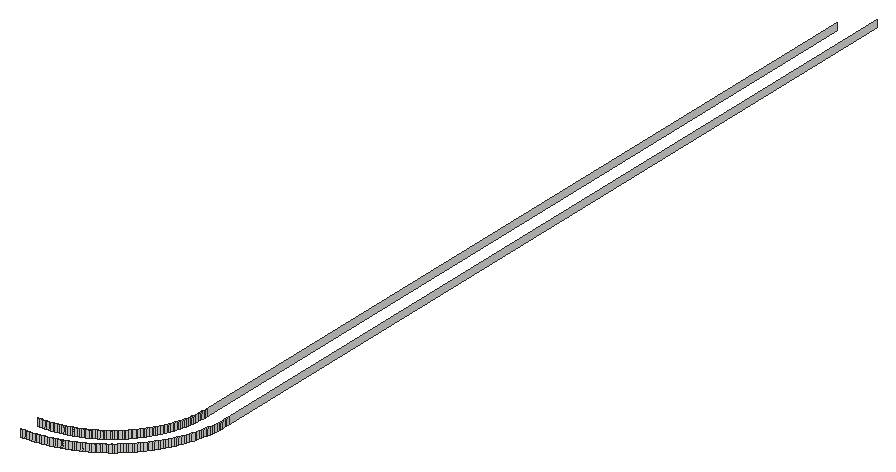
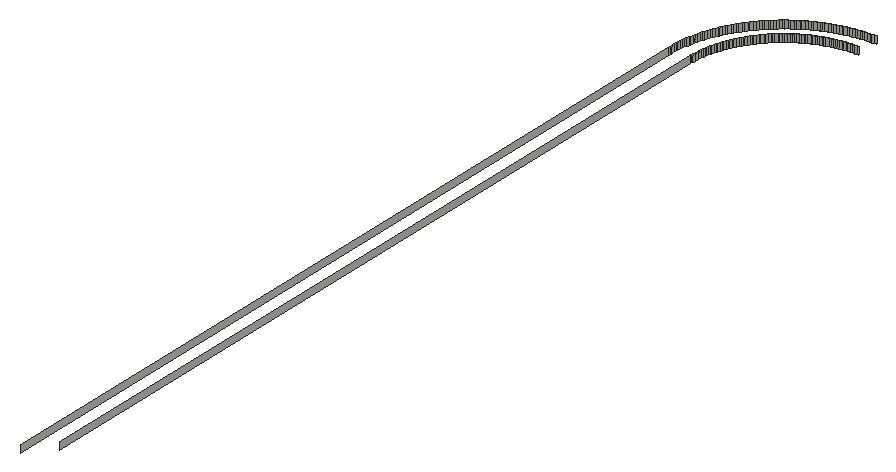
# SketchUp Ruby script. Lengths in inches.
U = 1.inch
M = Sketchup.active_model
def pt(a) = Geom::Point3d.new(a.map { |v| v * U })
def face(e, loops, mat)
  f = e.add_face(loops[0].map { |a| pt(a) })
  loops[1..].each { |l| e.add_face(l.map { |a| pt(a) }).erase! }
  f.material = f.back_material = mat if mat
  f
end
# faces: each face lists its corners as indices into pts; further lists are holes
def faces(e, pts, list, mat = nil) = list.each { |f| face(e, (f[0].is_a?(Array) ? f : [f]).map { |l| l.map { |i| pts[i] } }, mat) }
# xy, xz, yz: faces in a plane at the given z, y or x. An outline is a flat list of corners, or four numbers for a rectangle; further outlines are holes
def ring(l) = l.size == 4 ? [[l[0], l[1]], [l[2], l[1]], [l[2], l[3]], [l[0], l[3]]] : l.each_slice(2).to_a
def flat(e, list, mat, &to3) = list.each { |f| face(e, (f[0].is_a?(Array) ? f : [f]).map { |l| ring(l).map { |u, v| to3.(u, v) } }, mat) }
def xy(e, z, list, mat = nil) = flat(e, list, mat) { |x, y| [x, y, z] }
def xz(e, y, list, mat = nil) = flat(e, list, mat) { |x, z| [x, y, z] }
def yz(e, x, list, mat = nil) = flat(e, list, mat) { |y, z| [x, y, z] }
def lines(e, pts, list) = list.each { |a, b| e.add_line(pt(pts[a]), pt(pts[b])) }
# prism: a flat outline (further loops are holes) pulled along v
def prism(e, loops, v, mat = nil)
  f = face(e, loops, mat); d = Geom::Vector3d.new(v.map { |x| x * U })
  f.pushpull(f.normal.samedirection?(d) ? d.length : -d.length)
end
def box(e, o, s, mat = nil) = prism(e, [[o, [o[0] + s[0], o[1], o[2]], [o[0] + s[0], o[1] + s[1], o[2]], [o[0], o[1] + s[1], o[2]]]], [0, 0, s[2]], mat)
def at(x, y, z, deg = 0) = Geom::Transformation.translation(pt([x, y, z])) * Geom::Transformation.rotation(ORIGIN, Z_AXIS, deg.degrees)
def axes(o, x, y, z) = Geom::Transformation.new([*x, 0, *y, 0, *z, 0, *pt(o).to_a, 1])
def part(name) = M.definitions.add(name)
# library, detail: a bought-in or finely detailed component or shape, given as its bounding box
def library(name, o, s) = part(name).tap { |d| box(d.entities, o, s) }
def detail(e, o, s) = box(e.add_group.entities, o, s)
def put(e, d, t, mat = nil) = e.add_instance(d, t).tap { |i| i.material = mat if mat }
def group(e, t, mat = nil) = e.add_group.tap { |g| g.transformation = t; g.material = mat if mat }.entities
root = M.entities
xz(root,124,[[278,116,278.16,116.5]])
xz(root,124.01,[[278.3125,116,278.47,116.5]])
xz(root,125.5,[[278,116,278.13,116.5]])
xz(root,125.51,[[278.26,116,278.38,116.5]])
yz(root,284.49,[[131.62,116,131.74,116.5]])
yz(root,284.5,[[131.87,116,132,116.5],[132,116,186.5,116.5]])
yz(root,285.99,[[131.53,116,131.6875,116.5]])
yz(root,286,[[131.84,116,132,116.5],[132,116,188,116.5]])
p = [[278.3125,124.01,116],[278.16,124,116],[278.16,124,116.5],[278.3125,124.01,116.5],[278.63,124.02,116],[278.47,124.01,116],
  [278.47,124.01,116.5],[278.63,124.02,116.5],[278.78,124.04,116],[278.78,124.04,116.5],[278.94,124.06,116],[278.94,124.06,116.5],
  [279.1,124.08,116],[279.1,124.08,116.5],[279.25,124.1,116],[279.25,124.1,116.5],[279.41,124.125,116],[279.41,124.125,116.5],
  [279.5625,124.15,116],[279.5625,124.15,116.5],[279.71,124.1875,116],[279.71,124.1875,116.5],[279.87,124.22,116],[279.87,124.22,116.5],
  [280.02,124.26,116],[280.02,124.26,116.5],[280.17,124.3,116],[280.17,124.3,116.5],[280.32,124.34,116],[280.32,124.34,116.5],
  [280.47,124.39,116],[280.47,124.39,116.5],[280.62,124.44,116],[280.62,124.44,116.5],[280.77,124.49,116],[280.77,124.49,116.5],
  [280.92,124.55,116],[280.92,124.55,116.5],[281.0625,124.61,116],[281.0625,124.61,116.5],[281.21,124.67,116],[281.21,124.67,116.5],
  [281.35,124.73,116],[281.35,124.73,116.5],[281.49,124.8,116],[281.49,124.8,116.5],[281.63,124.87,116],[281.63,124.87,116.5],
  [281.77,124.94,116],[281.77,124.94,116.5],[281.91,125.02,116],[281.91,125.02,116.5],[282.05,125.1,116],[282.05,125.1,116.5],
  [282.18,125.18,116],[282.18,125.18,116.5],[282.3125,125.26,116],[282.3125,125.26,116.5],[282.44,125.35,116],[282.44,125.35,116.5],
  [282.57,125.4375,116],[282.57,125.4375,116.5],[282.7,125.53,116],[282.7,125.53,116.5],[278.13,125.5,116],[278.26,125.51,116],
  [278.26,125.51,116.5],[278.13,125.5,116.5],[278.38,125.51,116],[278.51,125.52,116],[278.51,125.52,116.5],[278.38,125.51,116.5],
  [278.64,125.53,116],[278.64,125.53,116.5],[278.76,125.55,116],[278.76,125.55,116.5],[278.89,125.5625,116],[278.89,125.5625,116.5],
  [282.83,125.62,116],[282.83,125.62,116.5],[279.02,125.58,116],[279.02,125.58,116.5],[279.14,125.6,116],[279.14,125.6,116.5],
  [279.27,125.625,116],[279.27,125.625,116.5],[279.39,125.65,116],[279.39,125.65,116.5],[282.95,125.72,116],[282.95,125.72,116.5],
  [279.52,125.68,116],[279.52,125.68,116.5],[279.64,125.71,116],[279.64,125.71,116.5],[279.76,125.74,116],[279.76,125.74,116.5],
  [279.89,125.78,116],[279.89,125.78,116.5],[283.08,125.82,116],[283.08,125.82,116.5],[280.01,125.82,116],[280.01,125.82,116.5],
  [280.13,125.86,116],[280.13,125.86,116.5],[283.2,125.92,116],[283.2,125.92,116.5],[280.25,125.9,116],[280.25,125.9,116.5],
  [280.37,125.95,116],[280.37,125.95,116.5],[280.49,125.99,116],[280.49,125.99,116.5],[283.3125,126.02,116],[283.3125,126.02,116.5],
  [280.6,126.04,116],[280.6,126.04,116.5],[280.72,126.1,116],[280.72,126.1,116.5],[283.43,126.125,116],[283.43,126.125,116.5],
  [280.84,126.15,116],[280.84,126.15,116.5],[283.54,126.23,116],[283.54,126.23,116.5],[280.95,126.21,116],[280.95,126.21,116.5],
  [281.0625,126.27,116],[281.0625,126.27,116.5],[283.66,126.34,116],[283.66,126.34,116.5],[281.18,126.33,116],[281.18,126.33,116.5],
  [281.29,126.39,116],[281.29,126.39,116.5],[283.77,126.46,116],[283.77,126.46,116.5],[281.4,126.46,116],[281.4,126.46,116.5],
  [281.5,126.53,116],[281.5,126.53,116.5],[281.61,126.6,116],[281.61,126.6,116.5],[283.875,126.57,116],[283.875,126.57,116.5],
  [281.72,126.67,116],[281.72,126.67,116.5],[283.98,126.6875,116],[283.98,126.6875,116.5],[281.82,126.74,116],[281.82,126.74,116.5],
  [281.92,126.82,116],[281.92,126.82,116.5],[284.08,126.8,116],[284.08,126.8,116.5],[282.02,126.9,116],[282.02,126.9,116.5],
  [284.18,126.92,116],[284.18,126.92,116.5],[282.125,126.98,116],[282.125,126.98,116.5],[284.28,127.05,116],[284.28,127.05,116.5],
  [282.22,127.06,116],[282.22,127.06,116.5],[284.38,127.17,116],[284.38,127.17,116.5],[282.32,127.14,116],[282.32,127.14,116.5],
  [282.41,127.23,116],[282.41,127.23,116.5],[282.5,127.3125,116],[282.5,127.3125,116.5],[284.47,127.3,116],[284.47,127.3,116.5],
  [282.6,127.4,116],[282.6,127.4,116.5],[284.5625,127.43,116],[284.5625,127.43,116.5],[282.69,127.49,116],[282.69,127.49,116.5],
  [284.65,127.56,116],[284.65,127.56,116.5],[282.77,127.59,116],[282.77,127.59,116.5],[282.86,127.68,116],[282.86,127.68,116.5],
  [284.74,127.6875,116],[284.74,127.6875,116.5],[282.94,127.78,116],[282.94,127.78,116.5],[284.82,127.82,116],[284.82,127.82,116.5],
  [283.02,127.875,116],[283.02,127.875,116.5],[284.9,127.95,116],[284.9,127.95,116.5],[283.1,127.98,116],[283.1,127.98,116.5],
  [283.18,128.08,116],[283.18,128.08,116.5],[284.98,128.09,116],[284.98,128.09,116.5],[283.26,128.18,116],[283.26,128.18,116.5],
  [285.06,128.23,116],[285.06,128.23,116.5],[283.33,128.28,116],[283.33,128.28,116.5],[285.13,128.37,116],[285.13,128.37,116.5],
  [283.4,128.39,116],[283.4,128.39,116.5],[283.47,128.5,116],[283.47,128.5,116.5],[285.2,128.51,116],[285.2,128.51,116.5],
  [283.54,128.6,116],[283.54,128.6,116.5],[285.27,128.65,116],[285.27,128.65,116.5],[283.61,128.71,116],[283.61,128.71,116.5],
  [283.67,128.82,116],[283.67,128.82,116.5],[285.33,128.79,116],[285.33,128.79,116.5],[283.73,128.9375,116],[283.73,128.9375,116.5],
  [285.39,128.9375,116],[285.39,128.9375,116.5],[283.79,129.05,116],[283.79,129.05,116.5],[285.45,129.08,116],[285.45,129.08,116.5],
  [283.85,129.16,116],[283.85,129.16,116.5],[285.51,129.23,116],[285.51,129.23,116.5],[283.9,129.28,116],[283.9,129.28,116.5],
  [285.56,129.38,116],[285.56,129.38,116.5],[283.96,129.4,116],[283.96,129.4,116.5],[284.01,129.51,116],[284.01,129.51,116.5],
  [285.61,129.53,116],[285.61,129.53,116.5],[284.05,129.63,116],[284.05,129.63,116.5],[285.66,129.68,116],[285.66,129.68,116.5],
  [284.1,129.75,116],[284.1,129.75,116.5],[285.7,129.83,116],[285.7,129.83,116.5],[284.14,129.87,116],[284.14,129.87,116.5],
  [285.74,129.98,116],[285.74,129.98,116.5],[284.18,129.99,116],[284.18,129.99,116.5],[284.22,130.11,116],[284.22,130.11,116.5],
  [285.78,130.13,116],[285.78,130.13,116.5],[284.26,130.24,116],[284.26,130.24,116.5],[285.8125,130.29,116],[285.8125,130.29,116.5],
  [284.29,130.36,116],[284.29,130.36,116.5],[285.85,130.4375,116],[285.85,130.4375,116.5],[284.32,130.48,116],[284.32,130.48,116.5],
  [285.875,130.59,116],[285.875,130.59,116.5],[284.35,130.61,116],[284.35,130.61,116.5],[284.375,130.73,116],[284.375,130.73,116.5],
  [285.9,130.75,116],[285.9,130.75,116.5],[284.4,130.86,116],[284.4,130.86,116.5],[285.92,130.9,116],[285.92,130.9,116.5],
  [284.42,130.98,116],[284.42,130.98,116.5],[285.94,131.06,116],[285.94,131.06,116.5],[284.4375,131.11,116],[284.4375,131.11,116.5],
  [284.45,131.24,116],[284.45,131.24,116.5],[285.96,131.22,116],[285.96,131.22,116.5],[284.47,131.36,116],[284.47,131.36,116.5],
  [285.98,131.37,116],[285.98,131.37,116.5],[284.48,131.49,116],[284.48,131.49,116.5],[285.99,131.53,116],[285.99,131.53,116.5],
  [284.49,131.62,116],[284.49,131.62,116.5],[284.49,131.74,116],[284.5,131.87,116],[284.5,131.87,116.5],[284.49,131.74,116.5],
  [286,131.84,116],[285.99,131.6875,116],[285.99,131.6875,116.5],[286,131.84,116.5]]
faces(root,p,[[0,1,2,3],[4,5,6,7],[8,4,7,9],[10,8,9,11],[12,10,11,13],[14,12,13,15],[16,14,15,17],[18,16,17,19],
  [20,18,19,21],[22,20,21,23],[24,22,23,25],[26,24,25,27],[28,26,27,29],[30,28,29,31],[32,30,31,33],[34,32,33,35],
  [36,34,35,37],[38,36,37,39],[40,38,39,41],[42,40,41,43],[44,42,43,45],[46,44,45,47],[48,46,47,49],[50,48,49,51],
  [52,50,51,53],[54,52,53,55],[56,54,55,57],[58,56,57,59],[60,58,59,61],[62,60,61,63],[64,65,66,67],[68,69,70,71],
  [69,72,73,70],[72,74,75,73],[74,76,77,75],[78,62,63,79],[76,80,81,77],[80,82,83,81],[82,84,85,83],[84,86,87,85],
  [88,78,79,89],[86,90,91,87],[90,92,93,91],[92,94,95,93],[94,96,97,95],[98,88,89,99],[96,100,101,97],[100,102,103,101],
  [104,98,99,105],[102,106,107,103],[106,108,109,107],[108,110,111,109],[112,104,105,113],[110,114,115,111],[114,116,117,115],[118,112,113,119],
  [116,120,121,117],[122,118,119,123],[120,124,125,121],[124,126,127,125],[128,122,123,129],[126,130,131,127],[130,132,133,131],[134,128,129,135],
  [132,136,137,133],[136,138,139,137],[138,140,141,139],[142,134,135,143],[140,144,145,141],[146,142,143,147],[144,148,149,145],[148,150,151,149],
  [152,146,147,153],[150,154,155,151],[156,152,153,157],[154,158,159,155],[160,156,157,161],[158,162,163,159],[164,160,161,165],[162,166,167,163],
  [166,168,169,167],[168,170,171,169],[172,164,165,173],[170,174,175,171],[176,172,173,177],[174,178,179,175],[180,176,177,181],[178,182,183,179],
  [182,184,185,183],[186,180,181,187],[184,188,189,185],[190,186,187,191],[188,192,193,189],[194,190,191,195],[192,196,197,193],[196,198,199,197],
  [200,194,195,201],[198,202,203,199],[204,200,201,205],[202,206,207,203],[208,204,205,209],[206,210,211,207],[210,212,213,211],[214,208,209,215],
  [212,216,217,213],[218,214,215,219],[216,220,221,217],[220,222,223,221],[224,218,219,225],[222,226,227,223],[228,224,225,229],[226,230,231,227],
  [232,228,229,233],[230,234,235,231],[236,232,233,237],[234,238,239,235],[240,236,237,241],[238,242,243,239],[242,244,245,243],[246,240,241,247],
  [244,248,249,245],[250,246,247,251],[248,252,253,249],[254,250,251,255],[252,256,257,253],[258,254,255,259],[256,260,261,257],[260,262,263,261],
  [264,258,259,265],[262,266,267,263],[268,264,265,269],[266,270,271,267],[272,268,269,273],[270,274,275,271],[276,272,273,277],[274,278,279,275],
  [278,280,281,279],[282,276,277,283],[280,284,285,281],[286,282,283,287],[284,288,289,285],[290,286,287,291],[288,292,293,289],[292,294,295,293],
  [296,290,291,297],[294,298,299,295],[300,296,297,301],[298,302,303,299],[304,300,301,305],[302,306,307,303],[308,309,310,311],[312,313,314,315]])
